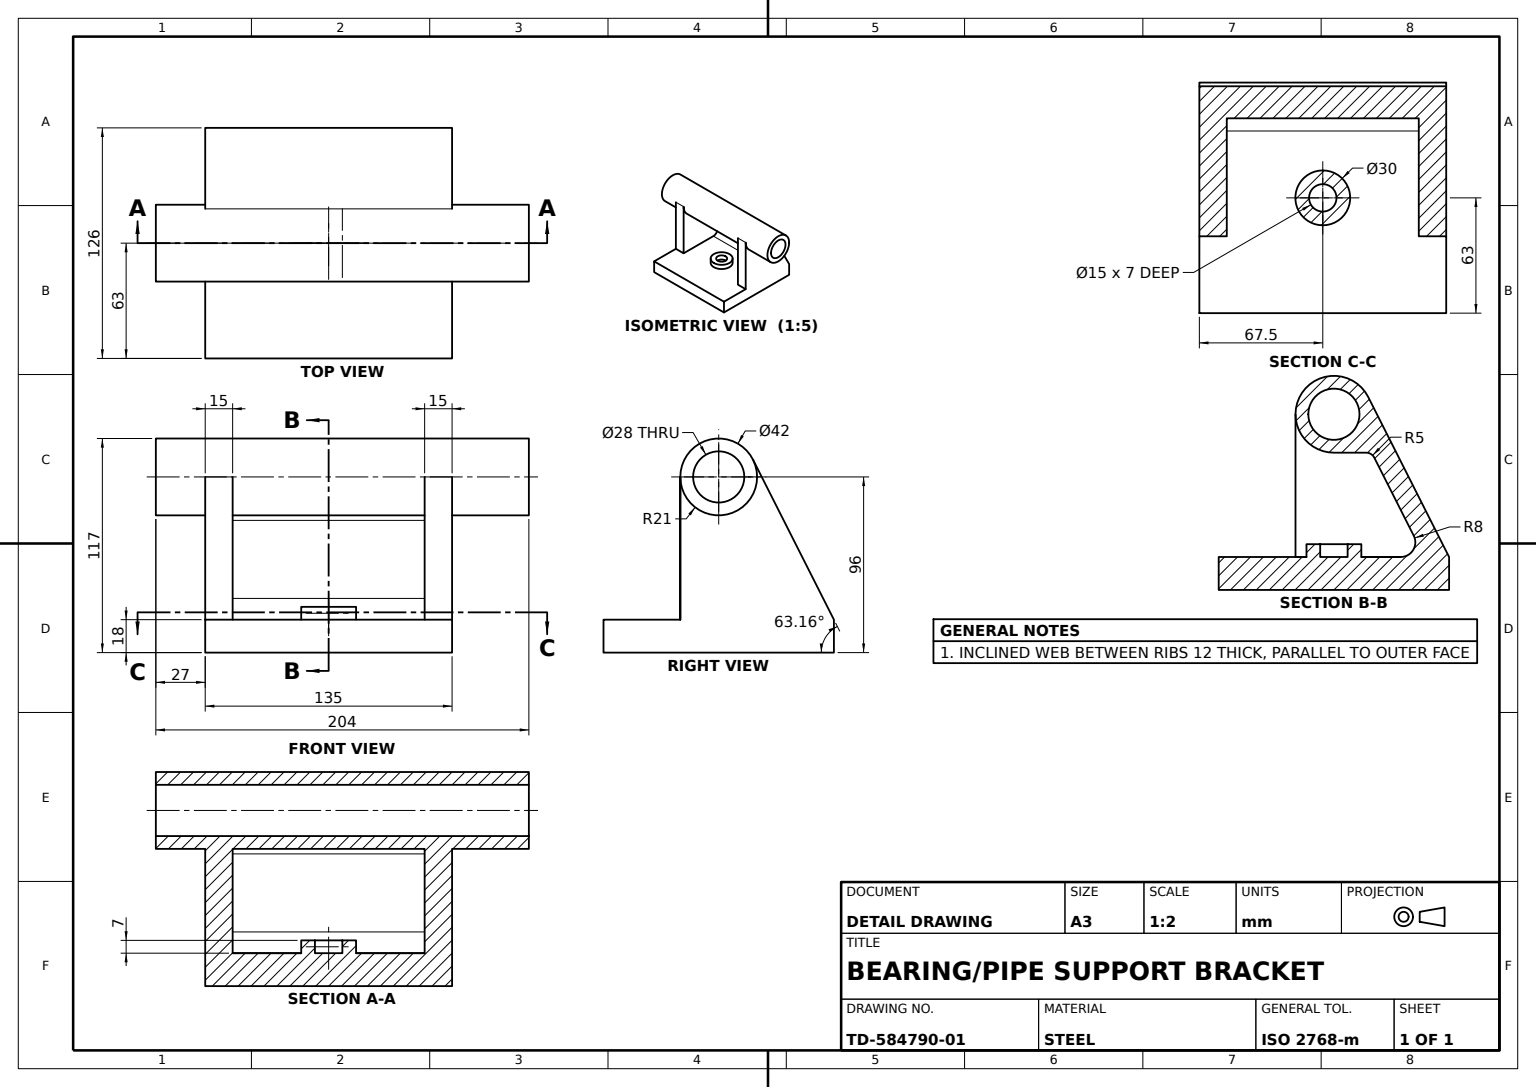
ISO-10303-21;
HEADER;
FILE_DESCRIPTION((''),'2;1');
FILE_NAME('','',(''),(''),'','','');
FILE_SCHEMA(('AUTOMOTIVE_DESIGN'));
ENDSEC;
DATA;
#1=APPLICATION_CONTEXT('');
#2=PRODUCT_CONTEXT('',#1,'mechanical');
#3=PRODUCT('','','',(#2));
#4=PRODUCT_DEFINITION_FORMATION('','',#3);
#5=PRODUCT_DEFINITION_CONTEXT('',#1,'design');
#6=PRODUCT_DEFINITION('','',#4,#5);
#7=PRODUCT_DEFINITION_SHAPE('','',#6);
#8=(LENGTH_UNIT()NAMED_UNIT(*)SI_UNIT(.MILLI.,.METRE.));
#9=(NAMED_UNIT(*)PLANE_ANGLE_UNIT()SI_UNIT($,.RADIAN.));
#10=(NAMED_UNIT(*)SI_UNIT($,.STERADIAN.)SOLID_ANGLE_UNIT());
#11=UNCERTAINTY_MEASURE_WITH_UNIT(LENGTH_MEASURE(1.E-05),#8,'distance_accuracy_value','');
#12=(GEOMETRIC_REPRESENTATION_CONTEXT(3)GLOBAL_UNCERTAINTY_ASSIGNED_CONTEXT((#11))GLOBAL_UNIT_ASSIGNED_CONTEXT((#8,#9,#10))REPRESENTATION_CONTEXT('',''));
#13=CARTESIAN_POINT('',(-52.5,75.,0.));
#14=VERTEX_POINT('',#13);
#15=CARTESIAN_POINT('',(-52.5,75.,-17.637861));
#16=VERTEX_POINT('',#15);
#17=DIRECTION('',(0.,0.,-1.));
#18=VECTOR('',#17,1000.);
#19=LINE('',#15,#18);
#20=EDGE_CURVE('',#14,#16,#19,.T.);
#21=ORIENTED_EDGE('',*,*,#20,.T.);
#22=CARTESIAN_POINT('',(52.5,75.,-17.637861));
#23=VERTEX_POINT('',#22);
#24=CARTESIAN_POINT('',(67.5,75.,-17.637861));
#25=DIRECTION('',(-1.,0.,0.));
#26=VECTOR('',#25,1000.);
#27=LINE('',#24,#26);
#28=EDGE_CURVE('',#23,#16,#27,.T.);
#29=ORIENTED_EDGE('',*,*,#28,.F.);
#30=CARTESIAN_POINT('',(52.5,75.,0.));
#31=VERTEX_POINT('',#30);
#32=DIRECTION('',(0.,0.,1.));
#33=VECTOR('',#32,1000.);
#34=LINE('',#22,#33);
#35=EDGE_CURVE('',#23,#31,#34,.T.);
#36=ORIENTED_EDGE('',*,*,#35,.T.);
#37=CARTESIAN_POINT('',(67.5,75.,0.));
#38=LINE('',#37,#26);
#39=EDGE_CURVE('',#31,#14,#38,.T.);
#40=ORIENTED_EDGE('',*,*,#39,.T.);
#41=EDGE_LOOP('',(#21,#29,#36,#40));
#42=FACE_OUTER_BOUND('',#41,.T.);
#43=DIRECTION('',(0.,1.,0.));
#44=AXIS2_PLACEMENT_3D('',#37,#43,#32);
#45=PLANE('',#44);
#46=ADVANCED_FACE('',(#42),#45,.F.);
#47=CARTESIAN_POINT('',(67.5,0.,63.));
#48=VERTEX_POINT('',#47);
#49=CARTESIAN_POINT('',(67.5,18.,63.));
#50=VERTEX_POINT('',#49);
#51=VECTOR('',#43,1000.);
#52=LINE('',#47,#51);
#53=EDGE_CURVE('',#48,#50,#52,.T.);
#54=ORIENTED_EDGE('',*,*,#53,.T.);
#55=CARTESIAN_POINT('',(-67.5,18.,63.));
#56=VERTEX_POINT('',#55);
#57=LINE('',#49,#26);
#58=EDGE_CURVE('',#50,#56,#57,.T.);
#59=ORIENTED_EDGE('',*,*,#58,.T.);
#60=CARTESIAN_POINT('',(-67.5,0.,63.));
#61=VERTEX_POINT('',#60);
#62=LINE('',#60,#51);
#63=EDGE_CURVE('',#61,#56,#62,.T.);
#64=ORIENTED_EDGE('',*,*,#63,.F.);
#65=LINE('',#47,#26);
#66=EDGE_CURVE('',#48,#61,#65,.T.);
#67=ORIENTED_EDGE('',*,*,#66,.F.);
#68=EDGE_LOOP('',(#54,#59,#64,#67));
#69=FACE_OUTER_BOUND('',#68,.T.);
#70=DIRECTION('',(1.,0.,0.));
#71=AXIS2_PLACEMENT_3D('',#47,#32,#70);
#72=PLANE('',#71);
#73=ADVANCED_FACE('',(#69),#72,.T.);
#74=CARTESIAN_POINT('',(-52.5,72.257322,-22.099307));
#75=VERTEX_POINT('',#74);
#76=CARTESIAN_POINT('',(-52.5,29.611715,-43.67636));
#77=VERTEX_POINT('',#76);
#78=DIRECTION('',(0.,-0.892289168,-0.451464328));
#79=VECTOR('',#78,1000.);
#80=LINE('',#76,#79);
#81=EDGE_CURVE('',#75,#77,#80,.T.);
#82=ORIENTED_EDGE('',*,*,#81,.T.);
#83=CARTESIAN_POINT('',(52.5,29.611715,-43.67636));
#84=VERTEX_POINT('',#83);
#85=CARTESIAN_POINT('',(67.5,29.611715,-43.67636));
#86=LINE('',#85,#26);
#87=EDGE_CURVE('',#84,#77,#86,.T.);
#88=ORIENTED_EDGE('',*,*,#87,.F.);
#89=CARTESIAN_POINT('',(52.5,72.257322,-22.099307));
#90=VERTEX_POINT('',#89);
#91=DIRECTION('',(0.,0.892289168,0.451464328));
#92=VECTOR('',#91,1000.);
#93=LINE('',#83,#92);
#94=EDGE_CURVE('',#84,#90,#93,.T.);
#95=ORIENTED_EDGE('',*,*,#94,.T.);
#96=CARTESIAN_POINT('',(67.5,72.257322,-22.099307));
#97=LINE('',#96,#26);
#98=EDGE_CURVE('',#90,#75,#97,.T.);
#99=ORIENTED_EDGE('',*,*,#98,.T.);
#100=EDGE_LOOP('',(#82,#88,#95,#99));
#101=FACE_OUTER_BOUND('',#100,.T.);
#102=CARTESIAN_POINT('',(67.5,23.629903,-46.702929));
#103=DIRECTION('',(0.,-0.451464328,0.892289168));
#104=AXIS2_PLACEMENT_3D('',#102,#103,#78);
#105=PLANE('',#104);
#106=ADVANCED_FACE('',(#101),#105,.T.);
#107=ORIENTED_EDGE('',*,*,#98,.F.);
#108=CARTESIAN_POINT('',(52.5,70.,-17.637861));
#109=AXIS2_PLACEMENT_3D('',#108,#70,#17);
#110=CIRCLE('',#109,5.);
#111=EDGE_CURVE('',#90,#23,#110,.T.);
#112=ORIENTED_EDGE('',*,*,#111,.T.);
#113=ORIENTED_EDGE('',*,*,#28,.T.);
#114=CARTESIAN_POINT('',(-52.5,70.,-17.637861));
#115=AXIS2_PLACEMENT_3D('',#114,#25,#17);
#116=CIRCLE('',#115,5.);
#117=EDGE_CURVE('',#16,#75,#116,.T.);
#118=ORIENTED_EDGE('',*,*,#117,.T.);
#119=EDGE_LOOP('',(#107,#112,#113,#118));
#120=FACE_OUTER_BOUND('',#119,.T.);
#121=CARTESIAN_POINT('',(67.5,70.,-17.637861));
#122=AXIS2_PLACEMENT_3D('',#121,#25,#32);
#123=CYLINDRICAL_SURFACE('',#122,5.);
#124=ADVANCED_FACE('',(#120),#123,.F.);
#125=CARTESIAN_POINT('',(-94.5,96.,-14.));
#126=VERTEX_POINT('',#125);
#127=CARTESIAN_POINT('',(-94.5,96.,14.));
#128=VERTEX_POINT('',#127);
#129=CARTESIAN_POINT('',(-94.5,96.,0.));
#130=AXIS2_PLACEMENT_3D('',#129,#25,#32);
#131=CIRCLE('',#130,14.);
#132=EDGE_CURVE('',#126,#128,#131,.T.);
#133=ORIENTED_EDGE('',*,*,#132,.F.);
#134=EDGE_CURVE('',#128,#126,#131,.T.);
#135=ORIENTED_EDGE('',*,*,#134,.F.);
#136=EDGE_LOOP('',(#133,#135));
#137=FACE_BOUND('',#136,.T.);
#138=CARTESIAN_POINT('',(-94.5,96.,21.));
#139=VERTEX_POINT('',#138);
#140=CARTESIAN_POINT('',(-94.5,96.,-21.));
#141=VERTEX_POINT('',#140);
#142=CIRCLE('',#130,21.);
#143=EDGE_CURVE('',#139,#141,#142,.T.);
#144=ORIENTED_EDGE('',*,*,#143,.T.);
#145=EDGE_CURVE('',#141,#139,#142,.T.);
#146=ORIENTED_EDGE('',*,*,#145,.T.);
#147=EDGE_LOOP('',(#144,#146));
#148=FACE_OUTER_BOUND('',#147,.T.);
#149=PLANE('',#130);
#150=ADVANCED_FACE('',(#137,#148),#149,.T.);
#151=CARTESIAN_POINT('',(109.5,96.,-14.));
#152=VERTEX_POINT('',#151);
#153=CARTESIAN_POINT('',(109.5,96.,14.));
#154=VERTEX_POINT('',#153);
#155=CARTESIAN_POINT('',(109.5,96.,0.));
#156=AXIS2_PLACEMENT_3D('',#155,#70,#17);
#157=CIRCLE('',#156,14.);
#158=EDGE_CURVE('',#152,#154,#157,.T.);
#159=ORIENTED_EDGE('',*,*,#158,.T.);
#160=CARTESIAN_POINT('',(67.5,96.,14.));
#161=LINE('',#160,#26);
#162=EDGE_CURVE('',#154,#128,#161,.T.);
#163=ORIENTED_EDGE('',*,*,#162,.T.);
#164=ORIENTED_EDGE('',*,*,#134,.T.);
#165=CARTESIAN_POINT('',(67.5,96.,-14.));
#166=LINE('',#165,#26);
#167=EDGE_CURVE('',#152,#126,#166,.T.);
#168=ORIENTED_EDGE('',*,*,#167,.F.);
#169=EDGE_LOOP('',(#159,#163,#164,#168));
#170=FACE_OUTER_BOUND('',#169,.T.);
#171=CARTESIAN_POINT('',(67.5,96.,0.));
#172=AXIS2_PLACEMENT_3D('',#171,#25,#32);
#173=CYLINDRICAL_SURFACE('',#172,14.);
#174=ADVANCED_FACE('',(#170),#173,.F.);
#175=CARTESIAN_POINT('',(52.5,96.,21.));
#176=VERTEX_POINT('',#175);
#177=CARTESIAN_POINT('',(52.5,96.,0.));
#178=AXIS2_PLACEMENT_3D('',#177,#25,#32);
#179=CIRCLE('',#178,21.);
#180=EDGE_CURVE('',#31,#176,#179,.T.);
#181=ORIENTED_EDGE('',*,*,#180,.T.);
#182=CARTESIAN_POINT('',(-52.5,96.,21.));
#183=VERTEX_POINT('',#182);
#184=CARTESIAN_POINT('',(67.5,96.,21.));
#185=LINE('',#184,#26);
#186=EDGE_CURVE('',#176,#183,#185,.T.);
#187=ORIENTED_EDGE('',*,*,#186,.T.);
#188=CARTESIAN_POINT('',(-52.5,96.,0.));
#189=AXIS2_PLACEMENT_3D('',#188,#70,#32);
#190=CIRCLE('',#189,21.);
#191=EDGE_CURVE('',#183,#14,#190,.T.);
#192=ORIENTED_EDGE('',*,*,#191,.T.);
#193=ORIENTED_EDGE('',*,*,#39,.F.);
#194=EDGE_LOOP('',(#181,#187,#192,#193));
#195=FACE_OUTER_BOUND('',#194,.T.);
#196=CYLINDRICAL_SURFACE('',#172,21.);
#197=ADVANCED_FACE('',(#195),#196,.T.);
#198=CARTESIAN_POINT('',(0.,18.,-7.5));
#199=VERTEX_POINT('',#198);
#200=CARTESIAN_POINT('',(0.,18.,7.5));
#201=VERTEX_POINT('',#200);
#202=CARTESIAN_POINT('',(0.,18.,0.));
#203=DIRECTION('',(0.,-1.,0.));
#204=AXIS2_PLACEMENT_3D('',#202,#203,#32);
#205=CIRCLE('',#204,7.5);
#206=EDGE_CURVE('',#199,#201,#205,.T.);
#207=ORIENTED_EDGE('',*,*,#206,.F.);
#208=EDGE_CURVE('',#201,#199,#205,.T.);
#209=ORIENTED_EDGE('',*,*,#208,.F.);
#210=EDGE_LOOP('',(#207,#209));
#211=FACE_OUTER_BOUND('',#210,.T.);
#212=CARTESIAN_POINT('',(67.5,18.,0.));
#213=AXIS2_PLACEMENT_3D('',#212,#43,#32);
#214=PLANE('',#213);
#215=ADVANCED_FACE('',(#211),#214,.T.);
#216=CARTESIAN_POINT('',(0.,25.,-15.));
#217=VERTEX_POINT('',#216);
#218=CARTESIAN_POINT('',(0.,18.,-15.));
#219=VERTEX_POINT('',#218);
#220=VECTOR('',#203,1000.);
#221=LINE('',#216,#220);
#222=EDGE_CURVE('',#217,#219,#221,.T.);
#223=ORIENTED_EDGE('',*,*,#222,.T.);
#224=CARTESIAN_POINT('',(0.,18.,15.));
#225=VERTEX_POINT('',#224);
#226=AXIS2_PLACEMENT_3D('',#202,#43,#32);
#227=CIRCLE('',#226,15.);
#228=EDGE_CURVE('',#219,#225,#227,.T.);
#229=ORIENTED_EDGE('',*,*,#228,.T.);
#230=CARTESIAN_POINT('',(0.,25.,15.));
#231=VERTEX_POINT('',#230);
#232=LINE('',#230,#220);
#233=EDGE_CURVE('',#231,#225,#232,.T.);
#234=ORIENTED_EDGE('',*,*,#233,.F.);
#235=CARTESIAN_POINT('',(0.,25.,0.));
#236=AXIS2_PLACEMENT_3D('',#235,#43,#32);
#237=CIRCLE('',#236,15.);
#238=EDGE_CURVE('',#217,#231,#237,.T.);
#239=ORIENTED_EDGE('',*,*,#238,.F.);
#240=EDGE_LOOP('',(#223,#229,#234,#239));
#241=FACE_OUTER_BOUND('',#240,.T.);
#242=AXIS2_PLACEMENT_3D('',#235,#203,#17);
#243=CYLINDRICAL_SURFACE('',#242,15.);
#244=ADVANCED_FACE('',(#241),#243,.T.);
#245=CARTESIAN_POINT('',(-67.5,96.,21.));
#246=VERTEX_POINT('',#245);
#247=EDGE_CURVE('',#246,#139,#185,.T.);
#248=ORIENTED_EDGE('',*,*,#247,.T.);
#249=ORIENTED_EDGE('',*,*,#145,.F.);
#250=CARTESIAN_POINT('',(-67.5,96.,-21.));
#251=VERTEX_POINT('',#250);
#252=CARTESIAN_POINT('',(67.5,96.,-21.));
#253=LINE('',#252,#26);
#254=EDGE_CURVE('',#251,#141,#253,.T.);
#255=ORIENTED_EDGE('',*,*,#254,.F.);
#256=CARTESIAN_POINT('',(-67.5,96.,0.));
#257=AXIS2_PLACEMENT_3D('',#256,#25,#32);
#258=CIRCLE('',#257,21.);
#259=EDGE_CURVE('',#251,#246,#258,.T.);
#260=ORIENTED_EDGE('',*,*,#259,.T.);
#261=EDGE_LOOP('',(#248,#249,#255,#260));
#262=FACE_OUTER_BOUND('',#261,.T.);
#263=ADVANCED_FACE('',(#262),#196,.T.);
#264=EDGE_CURVE('',#225,#219,#227,.T.);
#265=ORIENTED_EDGE('',*,*,#264,.F.);
#266=ORIENTED_EDGE('',*,*,#228,.F.);
#267=EDGE_LOOP('',(#265,#266));
#268=FACE_BOUND('',#267,.T.);
#269=CARTESIAN_POINT('',(52.5,18.,21.));
#270=VERTEX_POINT('',#269);
#271=CARTESIAN_POINT('',(52.5,18.,-36.538046));
#272=VERTEX_POINT('',#271);
#273=LINE('',#269,#18);
#274=EDGE_CURVE('',#270,#272,#273,.T.);
#275=ORIENTED_EDGE('',*,*,#274,.T.);
#276=CARTESIAN_POINT('',(-52.5,18.,-36.538046));
#277=VERTEX_POINT('',#276);
#278=CARTESIAN_POINT('',(67.5,18.,-36.538046));
#279=LINE('',#278,#26);
#280=EDGE_CURVE('',#272,#277,#279,.T.);
#281=ORIENTED_EDGE('',*,*,#280,.T.);
#282=CARTESIAN_POINT('',(-52.5,18.,21.));
#283=VERTEX_POINT('',#282);
#284=LINE('',#282,#33);
#285=EDGE_CURVE('',#277,#283,#284,.T.);
#286=ORIENTED_EDGE('',*,*,#285,.T.);
#287=CARTESIAN_POINT('',(-67.5,18.,21.));
#288=VERTEX_POINT('',#287);
#289=LINE('',#282,#26);
#290=EDGE_CURVE('',#283,#288,#289,.T.);
#291=ORIENTED_EDGE('',*,*,#290,.T.);
#292=CARTESIAN_POINT('',(-67.5,18.,0.));
#293=LINE('',#292,#18);
#294=EDGE_CURVE('',#56,#288,#293,.T.);
#295=ORIENTED_EDGE('',*,*,#294,.F.);
#296=ORIENTED_EDGE('',*,*,#58,.F.);
#297=CARTESIAN_POINT('',(67.5,18.,21.));
#298=VERTEX_POINT('',#297);
#299=LINE('',#212,#18);
#300=EDGE_CURVE('',#50,#298,#299,.T.);
#301=ORIENTED_EDGE('',*,*,#300,.T.);
#302=VECTOR('',#70,1000.);
#303=LINE('',#269,#302);
#304=EDGE_CURVE('',#270,#298,#303,.T.);
#305=ORIENTED_EDGE('',*,*,#304,.F.);
#306=EDGE_LOOP('',(#275,#281,#286,#291,#295,#296,#301,#305));
#307=FACE_OUTER_BOUND('',#306,.T.);
#308=ADVANCED_FACE('',(#268,#307),#214,.T.);
#309=CARTESIAN_POINT('',(67.5,0.,-63.));
#310=VERTEX_POINT('',#309);
#311=CARTESIAN_POINT('',(-67.5,0.,-63.));
#312=VERTEX_POINT('',#311);
#313=LINE('',#309,#26);
#314=EDGE_CURVE('',#310,#312,#313,.T.);
#315=ORIENTED_EDGE('',*,*,#314,.T.);
#316=CARTESIAN_POINT('',(-67.5,18.,-63.));
#317=VERTEX_POINT('',#316);
#318=LINE('',#311,#51);
#319=EDGE_CURVE('',#312,#317,#318,.T.);
#320=ORIENTED_EDGE('',*,*,#319,.T.);
#321=CARTESIAN_POINT('',(67.5,18.,-63.));
#322=VERTEX_POINT('',#321);
#323=LINE('',#321,#26);
#324=EDGE_CURVE('',#322,#317,#323,.T.);
#325=ORIENTED_EDGE('',*,*,#324,.F.);
#326=LINE('',#309,#51);
#327=EDGE_CURVE('',#310,#322,#326,.T.);
#328=ORIENTED_EDGE('',*,*,#327,.F.);
#329=EDGE_LOOP('',(#315,#320,#325,#328));
#330=FACE_OUTER_BOUND('',#329,.T.);
#331=AXIS2_PLACEMENT_3D('',#309,#32,#70);
#332=PLANE('',#331);
#333=ADVANCED_FACE('',(#330),#332,.F.);
#334=CARTESIAN_POINT('',(0.,25.,7.5));
#335=VERTEX_POINT('',#334);
#336=LINE('',#334,#220);
#337=EDGE_CURVE('',#335,#201,#336,.T.);
#338=ORIENTED_EDGE('',*,*,#337,.F.);
#339=CARTESIAN_POINT('',(0.,25.,-7.5));
#340=VERTEX_POINT('',#339);
#341=CIRCLE('',#236,7.5);
#342=EDGE_CURVE('',#335,#340,#341,.T.);
#343=ORIENTED_EDGE('',*,*,#342,.T.);
#344=LINE('',#339,#220);
#345=EDGE_CURVE('',#340,#199,#344,.T.);
#346=ORIENTED_EDGE('',*,*,#345,.T.);
#347=ORIENTED_EDGE('',*,*,#206,.T.);
#348=EDGE_LOOP('',(#338,#343,#346,#347));
#349=FACE_OUTER_BOUND('',#348,.T.);
#350=CYLINDRICAL_SURFACE('',#242,7.5);
#351=ADVANCED_FACE('',(#349),#350,.F.);
#352=ORIENTED_EDGE('',*,*,#132,.T.);
#353=ORIENTED_EDGE('',*,*,#162,.F.);
#354=EDGE_CURVE('',#154,#152,#157,.T.);
#355=ORIENTED_EDGE('',*,*,#354,.T.);
#356=ORIENTED_EDGE('',*,*,#167,.T.);
#357=EDGE_LOOP('',(#352,#353,#355,#356));
#358=FACE_OUTER_BOUND('',#357,.T.);
#359=ADVANCED_FACE('',(#358),#173,.F.);
#360=LINE('',#182,#26);
#361=EDGE_CURVE('',#183,#246,#360,.T.);
#362=ORIENTED_EDGE('',*,*,#361,.T.);
#363=LINE('',#245,#51);
#364=EDGE_CURVE('',#288,#246,#363,.T.);
#365=ORIENTED_EDGE('',*,*,#364,.F.);
#366=ORIENTED_EDGE('',*,*,#290,.F.);
#367=LINE('',#182,#51);
#368=EDGE_CURVE('',#283,#183,#367,.T.);
#369=ORIENTED_EDGE('',*,*,#368,.T.);
#370=EDGE_LOOP('',(#362,#365,#366,#369));
#371=FACE_OUTER_BOUND('',#370,.T.);
#372=AXIS2_PLACEMENT_3D('',#182,#32,#70);
#373=PLANE('',#372);
#374=ADVANCED_FACE('',(#371),#373,.T.);
#375=CARTESIAN_POINT('',(-67.5,105.480751,-18.738073));
#376=VERTEX_POINT('',#375);
#377=CARTESIAN_POINT('',(-67.5,29.047475,-57.410399));
#378=LINE('',#377,#92);
#379=EDGE_CURVE('',#317,#376,#378,.T.);
#380=ORIENTED_EDGE('',*,*,#379,.T.);
#381=CARTESIAN_POINT('',(67.5,105.480751,-18.738073));
#382=VERTEX_POINT('',#381);
#383=LINE('',#381,#26);
#384=EDGE_CURVE('',#382,#376,#383,.T.);
#385=ORIENTED_EDGE('',*,*,#384,.F.);
#386=CARTESIAN_POINT('',(67.5,29.047475,-57.410399));
#387=LINE('',#386,#92);
#388=EDGE_CURVE('',#322,#382,#387,.T.);
#389=ORIENTED_EDGE('',*,*,#388,.F.);
#390=ORIENTED_EDGE('',*,*,#324,.T.);
#391=EDGE_LOOP('',(#380,#385,#389,#390));
#392=FACE_OUTER_BOUND('',#391,.T.);
#393=AXIS2_PLACEMENT_3D('',#386,#103,#78);
#394=PLANE('',#393);
#395=ADVANCED_FACE('',(#392),#394,.F.);
#396=ORIENTED_EDGE('',*,*,#280,.F.);
#397=CARTESIAN_POINT('',(52.5,26.,-36.538046));
#398=AXIS2_PLACEMENT_3D('',#397,#70,#17);
#399=CIRCLE('',#398,8.);
#400=EDGE_CURVE('',#272,#84,#399,.T.);
#401=ORIENTED_EDGE('',*,*,#400,.T.);
#402=ORIENTED_EDGE('',*,*,#87,.T.);
#403=CARTESIAN_POINT('',(-52.5,26.,-36.538046));
#404=AXIS2_PLACEMENT_3D('',#403,#25,#17);
#405=CIRCLE('',#404,8.);
#406=EDGE_CURVE('',#77,#277,#405,.T.);
#407=ORIENTED_EDGE('',*,*,#406,.T.);
#408=EDGE_LOOP('',(#396,#401,#402,#407));
#409=FACE_OUTER_BOUND('',#408,.T.);
#410=CARTESIAN_POINT('',(67.5,26.,-36.538046));
#411=AXIS2_PLACEMENT_3D('',#410,#25,#32);
#412=CYLINDRICAL_SURFACE('',#411,8.);
#413=ADVANCED_FACE('',(#409),#412,.F.);
#414=ORIENTED_EDGE('',*,*,#238,.T.);
#415=EDGE_CURVE('',#231,#217,#237,.T.);
#416=ORIENTED_EDGE('',*,*,#415,.T.);
#417=EDGE_LOOP('',(#414,#416));
#418=FACE_OUTER_BOUND('',#417,.T.);
#419=EDGE_CURVE('',#340,#335,#341,.T.);
#420=ORIENTED_EDGE('',*,*,#419,.F.);
#421=ORIENTED_EDGE('',*,*,#342,.F.);
#422=EDGE_LOOP('',(#420,#421));
#423=FACE_BOUND('',#422,.T.);
#424=PLANE('',#236);
#425=ADVANCED_FACE('',(#418,#423),#424,.T.);
#426=CARTESIAN_POINT('',(-67.5,0.,0.));
#427=LINE('',#426,#18);
#428=EDGE_CURVE('',#61,#312,#427,.T.);
#429=ORIENTED_EDGE('',*,*,#428,.F.);
#430=ORIENTED_EDGE('',*,*,#63,.T.);
#431=ORIENTED_EDGE('',*,*,#294,.T.);
#432=ORIENTED_EDGE('',*,*,#364,.T.);
#433=ORIENTED_EDGE('',*,*,#259,.F.);
#434=EDGE_CURVE('',#376,#251,#258,.T.);
#435=ORIENTED_EDGE('',*,*,#434,.F.);
#436=ORIENTED_EDGE('',*,*,#379,.F.);
#437=ORIENTED_EDGE('',*,*,#319,.F.);
#438=EDGE_LOOP('',(#429,#430,#431,#432,#433,#435,#436,#437));
#439=FACE_OUTER_BOUND('',#438,.T.);
#440=AXIS2_PLACEMENT_3D('',#426,#70,#17);
#441=PLANE('',#440);
#442=ADVANCED_FACE('',(#439),#441,.F.);
#443=ORIENTED_EDGE('',*,*,#111,.F.);
#444=ORIENTED_EDGE('',*,*,#94,.F.);
#445=ORIENTED_EDGE('',*,*,#400,.F.);
#446=ORIENTED_EDGE('',*,*,#274,.F.);
#447=LINE('',#175,#220);
#448=EDGE_CURVE('',#176,#270,#447,.T.);
#449=ORIENTED_EDGE('',*,*,#448,.F.);
#450=ORIENTED_EDGE('',*,*,#180,.F.);
#451=ORIENTED_EDGE('',*,*,#35,.F.);
#452=EDGE_LOOP('',(#443,#444,#445,#446,#449,#450,#451));
#453=FACE_OUTER_BOUND('',#452,.T.);
#454=PLANE('',#178);
#455=ADVANCED_FACE('',(#453),#454,.T.);
#456=CARTESIAN_POINT('',(67.5,0.,0.));
#457=LINE('',#456,#18);
#458=EDGE_CURVE('',#48,#310,#457,.T.);
#459=ORIENTED_EDGE('',*,*,#458,.F.);
#460=ORIENTED_EDGE('',*,*,#66,.T.);
#461=ORIENTED_EDGE('',*,*,#428,.T.);
#462=ORIENTED_EDGE('',*,*,#314,.F.);
#463=EDGE_LOOP('',(#459,#460,#461,#462));
#464=FACE_OUTER_BOUND('',#463,.T.);
#465=AXIS2_PLACEMENT_3D('',#456,#43,#32);
#466=PLANE('',#465);
#467=ADVANCED_FACE('',(#464),#466,.F.);
#468=ORIENTED_EDGE('',*,*,#53,.F.);
#469=ORIENTED_EDGE('',*,*,#458,.T.);
#470=ORIENTED_EDGE('',*,*,#327,.T.);
#471=ORIENTED_EDGE('',*,*,#388,.T.);
#472=VERTEX_POINT('',#252);
#473=AXIS2_PLACEMENT_3D('',#171,#70,#17);
#474=CIRCLE('',#473,21.);
#475=EDGE_CURVE('',#472,#382,#474,.T.);
#476=ORIENTED_EDGE('',*,*,#475,.F.);
#477=VERTEX_POINT('',#184);
#478=EDGE_CURVE('',#477,#472,#474,.T.);
#479=ORIENTED_EDGE('',*,*,#478,.F.);
#480=LINE('',#184,#220);
#481=EDGE_CURVE('',#477,#298,#480,.T.);
#482=ORIENTED_EDGE('',*,*,#481,.T.);
#483=ORIENTED_EDGE('',*,*,#300,.F.);
#484=EDGE_LOOP('',(#468,#469,#470,#471,#476,#479,#482,#483));
#485=FACE_OUTER_BOUND('',#484,.T.);
#486=AXIS2_PLACEMENT_3D('',#456,#70,#17);
#487=PLANE('',#486);
#488=ADVANCED_FACE('',(#485),#487,.T.);
#489=CARTESIAN_POINT('',(109.5,96.,21.));
#490=VERTEX_POINT('',#489);
#491=CARTESIAN_POINT('',(109.5,96.,-21.));
#492=VERTEX_POINT('',#491);
#493=CIRCLE('',#156,21.);
#494=EDGE_CURVE('',#490,#492,#493,.T.);
#495=ORIENTED_EDGE('',*,*,#494,.F.);
#496=EDGE_CURVE('',#490,#477,#185,.T.);
#497=ORIENTED_EDGE('',*,*,#496,.T.);
#498=ORIENTED_EDGE('',*,*,#478,.T.);
#499=EDGE_CURVE('',#492,#472,#253,.T.);
#500=ORIENTED_EDGE('',*,*,#499,.F.);
#501=EDGE_LOOP('',(#495,#497,#498,#500));
#502=FACE_OUTER_BOUND('',#501,.T.);
#503=ADVANCED_FACE('',(#502),#196,.T.);
#504=ORIENTED_EDGE('',*,*,#304,.T.);
#505=ORIENTED_EDGE('',*,*,#481,.F.);
#506=LINE('',#175,#302);
#507=EDGE_CURVE('',#176,#477,#506,.T.);
#508=ORIENTED_EDGE('',*,*,#507,.F.);
#509=ORIENTED_EDGE('',*,*,#448,.T.);
#510=EDGE_LOOP('',(#504,#505,#508,#509));
#511=FACE_OUTER_BOUND('',#510,.T.);
#512=AXIS2_PLACEMENT_3D('',#175,#32,#203);
#513=PLANE('',#512);
#514=ADVANCED_FACE('',(#511),#513,.T.);
#515=ORIENTED_EDGE('',*,*,#345,.F.);
#516=ORIENTED_EDGE('',*,*,#419,.T.);
#517=ORIENTED_EDGE('',*,*,#337,.T.);
#518=ORIENTED_EDGE('',*,*,#208,.T.);
#519=EDGE_LOOP('',(#515,#516,#517,#518));
#520=FACE_OUTER_BOUND('',#519,.T.);
#521=ADVANCED_FACE('',(#520),#350,.F.);
#522=ORIENTED_EDGE('',*,*,#354,.F.);
#523=ORIENTED_EDGE('',*,*,#158,.F.);
#524=EDGE_LOOP('',(#522,#523));
#525=FACE_BOUND('',#524,.T.);
#526=ORIENTED_EDGE('',*,*,#494,.T.);
#527=EDGE_CURVE('',#492,#490,#493,.T.);
#528=ORIENTED_EDGE('',*,*,#527,.T.);
#529=EDGE_LOOP('',(#526,#528));
#530=FACE_OUTER_BOUND('',#529,.T.);
#531=PLANE('',#156);
#532=ADVANCED_FACE('',(#525,#530),#531,.T.);
#533=ORIENTED_EDGE('',*,*,#415,.F.);
#534=ORIENTED_EDGE('',*,*,#233,.T.);
#535=ORIENTED_EDGE('',*,*,#264,.T.);
#536=ORIENTED_EDGE('',*,*,#222,.F.);
#537=EDGE_LOOP('',(#533,#534,#535,#536));
#538=FACE_OUTER_BOUND('',#537,.T.);
#539=ADVANCED_FACE('',(#538),#243,.T.);
#540=ORIENTED_EDGE('',*,*,#434,.T.);
#541=ORIENTED_EDGE('',*,*,#254,.T.);
#542=ORIENTED_EDGE('',*,*,#143,.F.);
#543=ORIENTED_EDGE('',*,*,#247,.F.);
#544=ORIENTED_EDGE('',*,*,#361,.F.);
#545=ORIENTED_EDGE('',*,*,#186,.F.);
#546=ORIENTED_EDGE('',*,*,#507,.T.);
#547=ORIENTED_EDGE('',*,*,#496,.F.);
#548=ORIENTED_EDGE('',*,*,#527,.F.);
#549=ORIENTED_EDGE('',*,*,#499,.T.);
#550=ORIENTED_EDGE('',*,*,#475,.T.);
#551=ORIENTED_EDGE('',*,*,#384,.T.);
#552=EDGE_LOOP('',(#540,#541,#542,#543,#544,#545,#546,#547,#548,#549,#550,#551));
#553=FACE_OUTER_BOUND('',#552,.T.);
#554=ADVANCED_FACE('',(#553),#196,.T.);
#555=ORIENTED_EDGE('',*,*,#20,.F.);
#556=ORIENTED_EDGE('',*,*,#191,.F.);
#557=ORIENTED_EDGE('',*,*,#368,.F.);
#558=ORIENTED_EDGE('',*,*,#285,.F.);
#559=ORIENTED_EDGE('',*,*,#406,.F.);
#560=ORIENTED_EDGE('',*,*,#81,.F.);
#561=ORIENTED_EDGE('',*,*,#117,.F.);
#562=EDGE_LOOP('',(#555,#556,#557,#558,#559,#560,#561));
#563=FACE_OUTER_BOUND('',#562,.T.);
#564=AXIS2_PLACEMENT_3D('',#188,#25,#32);
#565=PLANE('',#564);
#566=ADVANCED_FACE('',(#563),#565,.F.);
#567=CLOSED_SHELL('',(#46,#73,#106,#124,#150,#174,#197,#215,#244,#263,#308,#333,#351,#359,#374,#395,#413,#425,#442,#455,#467,#488,#503,#514,#521,#532,#539,#554,#566));
#568=MANIFOLD_SOLID_BREP('',#567);
#569=ADVANCED_BREP_SHAPE_REPRESENTATION('',(#568),#12);
#570=SHAPE_DEFINITION_REPRESENTATION(#7,#569);
ENDSEC;
END-ISO-10303-21;
